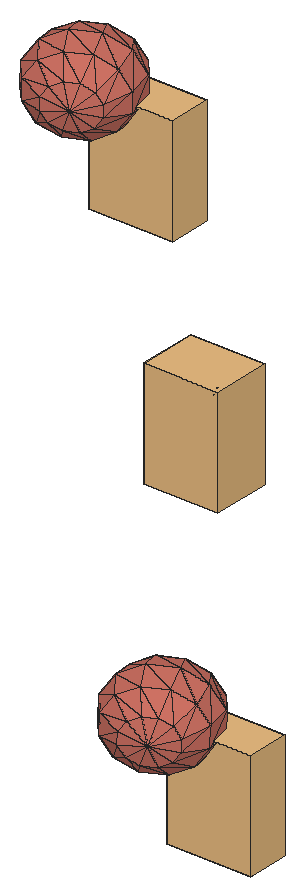
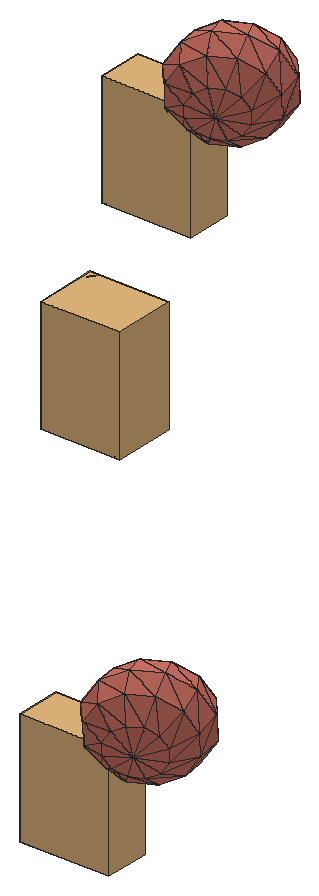
# SketchUp Ruby script. Lengths in inches.
U = 1.inch
M = Sketchup.active_model
def pt(a) = Geom::Point3d.new(a.map { |v| v * U })
def face(e, loops, mat)
  f = e.add_face(loops[0].map { |a| pt(a) })
  loops[1..].each { |l| e.add_face(l.map { |a| pt(a) }).erase! }
  f.material = f.back_material = mat if mat
  f
end
# faces: each face lists its corners as indices into pts; further lists are holes
def faces(e, pts, list, mat = nil) = list.each { |f| face(e, (f[0].is_a?(Array) ? f : [f]).map { |l| l.map { |i| pts[i] } }, mat) }
# xy, xz, yz: faces in a plane at the given z, y or x. An outline is a flat list of corners, or four numbers for a rectangle; further outlines are holes
def ring(l) = l.size == 4 ? [[l[0], l[1]], [l[2], l[1]], [l[2], l[3]], [l[0], l[3]]] : l.each_slice(2).to_a
def flat(e, list, mat, &to3) = list.each { |f| face(e, (f[0].is_a?(Array) ? f : [f]).map { |l| ring(l).map { |u, v| to3.(u, v) } }, mat) }
def xy(e, z, list, mat = nil) = flat(e, list, mat) { |x, y| [x, y, z] }
def xz(e, y, list, mat = nil) = flat(e, list, mat) { |x, z| [x, y, z] }
def yz(e, x, list, mat = nil) = flat(e, list, mat) { |y, z| [x, y, z] }
def lines(e, pts, list) = list.each { |a, b| e.add_line(pt(pts[a]), pt(pts[b])) }
# prism: a flat outline (further loops are holes) pulled along v
def prism(e, loops, v, mat = nil)
  f = face(e, loops, mat); d = Geom::Vector3d.new(v.map { |x| x * U })
  f.pushpull(f.normal.samedirection?(d) ? d.length : -d.length)
end
def box(e, o, s, mat = nil) = prism(e, [[o, [o[0] + s[0], o[1], o[2]], [o[0] + s[0], o[1] + s[1], o[2]], [o[0], o[1] + s[1], o[2]]]], [0, 0, s[2]], mat)
def at(x, y, z, deg = 0) = Geom::Transformation.translation(pt([x, y, z])) * Geom::Transformation.rotation(ORIGIN, Z_AXIS, deg.degrees)
def axes(o, x, y, z) = Geom::Transformation.new([*x, 0, *y, 0, *z, 0, *pt(o).to_a, 1])
def part(name) = M.definitions.add(name)
# library, detail: a bought-in or finely detailed component or shape, given as its bounding box
def library(name, o, s) = part(name).tap { |d| box(d.entities, o, s) }
def detail(e, o, s) = box(e.add_group.entities, o, s)
def put(e, d, t, mat = nil) = e.add_instance(d, t).tap { |i| i.material = mat if mat }
def group(e, t, mat = nil) = e.add_group.tap { |g| g.transformation = t; g.material = mat if mat }.entities
root = M.entities
M.materials.add("green").color = [174, 139, 102]
M.materials.add("vio").color = [206, 114, 100]
c1 = part("3DGeom~219_Defintion")
p = [[167.16,-297.35,-320.32],[-80.93,-262.73,-388.47],[-36.76,-95.49,-489.125],[218.17,-104.25,-436.54],[-281.83,-61.15,-410.64],[-43.21,95.93,-488.48],
  [-285.56,49.37,-410.27],[210.71,116.79,-435.8],[-317.52,144.24,-351.51],[-98.5625,260.26,-386.7],[-98.5625,260.26,-386.7],[370.46,-252.3,-166.34],
  [370.46,-252.3,-166.34],[414.63,-85.07,-266.99],[414.63,-85.07,-266.99],[414.63,-85.07,-266.99],[408.18,106.36,-266.34],[408.18,106.36,-266.34],
  [146.8,306.54,-318.28],[-98.5625,260.26,-386.7],[146.8,306.54,-318.28],[-307.34,-157.7,-352.53],[-281.83,-61.15,-410.64],[-307.34,-157.7,-352.53],
  [-451.39,-10.42,-222.13],[-285.56,49.37,-410.27],[-281.83,-61.15,-410.64],[-317.52,144.24,-351.51],[-285.56,49.37,-410.27],[71.36,-410.78,-118.27],
  [-163.89,-360.96,-213.49],[-80.93,-262.73,-388.47],[-80.93,-262.73,-388.47],[167.16,-297.35,-320.32],[-163.89,-360.96,-213.49],[-98.5625,260.26,-386.7],
  [-369.14,198.04,-250.11],[-98.5625,260.26,-386.7],[-369.14,198.04,-250.11],[-187.98,353.45,-211.07],[146.8,306.54,-318.28],[-98.5625,260.26,-386.7],
  [-187.98,353.45,-211.07],[-163.89,-360.96,-213.49],[-355.23,-214.42,-251.51],[-307.34,-157.7,-352.53],[-355.23,-214.42,-251.51],[-369.14,198.04,-250.11],
  [-317.52,144.24,-351.51],[287.5,-350.53,8.64],[167.16,-297.35,-320.32],[287.5,-350.53,8.64],[167.16,-297.35,-320.32],[370.46,-252.3,-166.34],
  [408.18,106.36,-266.34],[146.8,306.54,-318.28],[352.83,270.68,-164.57],[352.83,270.68,-164.57],[43.55,414.14,-115.47],[474.5,-139.65,32.21],
  [370.46,-252.3,-166.34],[414.63,-85.07,-266.99],[500,-43.09,-25.9],[408.18,106.36,-266.34],[496.27,67.43,-25.53],[352.83,270.68,-164.57],
  [-263.41,-363.87,-11.0625],[-412.69,-216.1,-134.63],[-355.23,-214.42,-251.51],[-355.23,-214.42,-251.51],[-355.23,-214.42,-251.51],[-412.69,-216.1,-134.63],
  [-426.6,196.36,-133.24],[-187.98,353.45,-211.07],[-412.69,-216.1,-134.63],[-464.32,-162.3,-33.23],[-496.27,-67.42,25.53],[-500,43.09,25.9],
  [-474.5,139.65,-32.21],[-43.55,-414.14,115.47],[-187.98,353.45,-211.07],[-287.5,350.54,-8.64],[-287.5,350.54,-8.64],[426.6,-196.36,133.24],
  [287.5,-350.53,8.64],[464.32,162.3,33.23],[263.41,363.87,11.0625],[352.83,270.68,-164.57],[263.41,363.87,11.0625],[-352.83,-270.68,164.57],
  [-412.69,-216.1,-134.63],[-263.41,-363.87,-11.0625],[-352.83,-270.68,164.57],[-412.69,-216.1,-134.63],[-287.5,350.54,-8.64],[187.98,-353.45,211.07],
  [187.98,-353.45,211.07],[287.5,-350.53,8.64],[-71.36,410.78,118.27],[-408.18,-106.36,266.34],[-352.83,-270.68,164.57],[-408.18,-106.36,266.34],
  [-370.46,252.3,166.34],[-287.5,350.54,-8.64],[-370.46,252.3,166.34],[451.39,10.42,222.13],[-146.8,-306.54,318.28],[-146.8,-306.54,318.28],
  [-352.83,-270.68,164.57],[-370.46,252.3,166.34],[369.14,-198.04,250.11],[187.98,-353.45,211.07],[263.41,363.87,11.0625],[412.69,216.1,134.63],
  [412.69,216.1,134.63],[163.89,360.96,213.49],[163.89,360.96,213.49],[-414.63,85.07,266.99],[-408.18,-106.36,266.34],[-414.63,85.07,266.99],
  [-370.46,252.3,166.34],[-414.63,85.07,266.99],[98.5625,-260.26,386.7],[-146.8,-306.54,318.28],[98.5625,-260.26,386.7],[187.98,-353.45,211.07],
  [-370.46,252.3,166.34],[-167.16,297.35,320.32],[163.89,360.96,213.49],[-167.16,297.35,320.32],[355.23,214.42,251.51],[412.69,216.1,134.63],
  [163.89,360.96,213.49],[355.23,214.42,251.51],[-210.71,-116.79,435.8],[-352.83,-270.68,164.57],[-146.8,-306.54,318.28],[-408.18,-106.36,266.34],
  [-167.16,297.35,320.32],[-370.46,252.3,166.34],[-414.63,85.07,266.99],[317.52,-144.24,351.51],[98.5625,-260.26,386.7],[187.98,-353.45,211.07],
  [317.52,-144.24,351.51],[187.98,-353.45,211.07],[369.14,-198.04,250.11],[355.23,214.42,251.51],[163.89,360.96,213.49],[80.93,262.73,388.47],
  [163.89,360.96,213.49],[-167.16,297.35,320.32],[80.93,262.73,388.47],[317.52,-144.24,351.51],[285.56,-49.37,410.27],[281.83,61.15,410.64],
  [307.34,157.7,352.53],[355.23,214.42,251.51],[307.34,157.7,352.53],[-218.17,104.25,436.54],[43.21,-95.93,488.48],[285.56,-49.37,410.27],
  [317.52,-144.24,351.51],[307.34,157.7,352.53],[36.76,95.49,489.125],[281.83,61.15,410.64],[307.34,157.7,352.53],[285.56,-49.37,410.27],
  [281.83,61.15,410.64],[285.56,-49.37,410.27],[281.83,61.15,410.64]]
faces(c1.entities,p,[[0,1,2],[0,2,3],[1,4,2],[3,2,5],[2,4,6],[2,6,5],[3,5,7],[5,6,8],
  [5,8,9],[7,5,10],[11,0,3],[12,3,13],[14,3,7],[15,7,16],[17,7,18],[7,19,20],
  [1,21,4],[22,23,24],[25,26,24],[27,28,24],[29,30,31],[29,32,33],[34,21,1],[35,8,36],
  [37,38,39],[40,41,42],[43,44,21],[45,46,24],[47,48,24],[49,29,50],[51,52,53],[54,55,56],
  [57,40,58],[40,42,58],[59,60,61],[59,61,62],[62,61,63],[62,63,64],[64,63,65],[66,67,68],
  [66,69,30],[70,71,24],[72,47,24],[73,47,72],[74,75,24],[75,76,24],[76,77,24],[77,78,24],
  [78,72,24],[79,66,30],[79,30,29],[80,72,81],[58,42,82],[83,84,60],[83,60,59],[64,65,85],
  [85,65,86],[87,58,88],[89,90,91],[92,75,93],[94,72,78],[95,79,29],[96,29,97],[58,82,98],
  [88,58,98],[99,75,100],[101,76,75],[102,78,77],[103,78,104],[59,62,105],[62,64,105],[64,85,105],
  [106,66,79],[107,108,66],[98,82,109],[110,111,84],[110,84,83],[85,112,113],[114,88,115],[88,98,116],
  [117,76,118],[119,77,76],[120,77,121],[83,59,105],[85,113,105],[122,123,79],[124,79,125],[98,126,127],
  [128,98,129],[110,83,105],[113,130,105],[131,132,133],[134,135,136],[134,137,135],[138,139,140],[141,142,143],
  [144,145,146],[147,148,149],[150,151,152],[153,110,105],[154,153,105],[155,154,105],[156,155,105],[130,156,105],
  [157,149,158],[159,137,134],[159,140,137],[138,140,159],[160,134,136],[160,136,142],[149,138,159],[161,142,162],
  [163,164,165],[166,149,164],[167,160,142],[149,159,164],[168,160,169],[170,164,160],[164,159,134],[164,134,160]],"vio")
c2 = library("3DGeom~96_Defintion",[-195.05,-500,-388.01],[390.1,1000,776.02])
c3 = part("3DGeom~97_Defintion")
p = [[174.48,487.39,-384.2],[155.8125,487.85,-388.01],[137.83,489.88,-382.14],[174.48,487.39,-384.2],[125.36,492.93,-368.18],[121.74,496.1875,-349.85],
  [174.48,487.39,-384.2],[121.74,496.1875,-349.85],[127.94,498.77,-332.09],[174.48,487.39,-384.2],[137.83,489.88,-382.14],[125.36,492.93,-368.18],
  [174.48,487.39,-384.2],[127.94,498.77,-332.09],[142.3,500,-319.63],[174.48,487.39,-384.2],[142.3,500,-319.63],[160.98,499.54,-315.83],
  [174.48,487.39,-384.2],[160.98,499.54,-315.83],[178.96,497.51,-321.7],[174.48,487.39,-384.2],[191.43,494.46,-335.66],[195.05,491.2,-353.98],
  [174.48,487.39,-384.2],[195.05,491.2,-353.98],[188.85,488.61,-371.75],[174.48,487.39,-384.2],[178.96,497.51,-321.7],[191.43,494.46,-335.66],
  [-147.29,-500,333.96],[-182.28,-490.37,332.19],[-165.51,-497.625,329.13],[-182.28,-490.37,332.19],[-147.29,-500,333.96],[-195.05,-469.79,356.79],
  [-182.28,-490.37,332.19],[-195.05,-469.79,356.79],[-193.09,-480.18,342.3125],[-195.05,-469.79,356.79],[-147.29,-500,333.96],[-172.82,-458.84,383.18],
  [-172.82,-458.84,383.18],[-147.29,-500,333.96],[-137.83,-468.47,384.95],[-147.29,-500,333.96],[-132.48,-496.86,345.39],[-125.0625,-489.05,360.34],
  [-137.83,-468.47,384.95],[-147.29,-500,333.96],[-125.0625,-489.05,360.34],[-195.05,-469.79,356.79],[-172.82,-458.84,383.18],[-187.63,-461.98,371.75],
  [-137.83,-468.47,384.95],[-125.0625,-489.05,360.34],[-127.02,-478.66,374.83],[-172.82,-458.84,383.18],[-137.83,-468.47,384.95],[-154.59,-461.21,388.01]]
faces(c3.entities,p,[[0,1,2],[3,4,5],[6,7,8],[9,10,11],[12,13,14],[15,16,17],[18,19,20],[21,22,23],
  [24,25,26],[27,28,29],[30,31,32],[33,34,35],[36,37,38],[39,40,41],[42,43,44],[45,46,47],
  [48,49,50],[51,52,53],[54,55,56],[57,58,59]],"green")
c4 = part("3DGeom~218_Defintion")
p = [[167.16,-297.35,-320.32],[-80.93,-262.73,-388.47],[-36.76,-95.49,-489.125],[218.17,-104.25,-436.54],[-281.83,-61.15,-410.64],[-43.21,95.93,-488.48],
  [-285.56,49.37,-410.27],[210.71,116.79,-435.8],[-317.52,144.24,-351.51],[-98.5625,260.26,-386.7],[-98.5625,260.26,-386.7],[370.46,-252.3,-166.34],
  [370.46,-252.3,-166.34],[414.63,-85.07,-266.99],[414.63,-85.07,-266.99],[414.63,-85.07,-266.99],[408.18,106.36,-266.34],[408.18,106.36,-266.34],
  [146.8,306.54,-318.28],[-98.5625,260.26,-386.7],[146.8,306.54,-318.28],[-307.34,-157.7,-352.53],[-281.83,-61.15,-410.64],[-307.34,-157.7,-352.53],
  [-451.39,-10.42,-222.13],[-285.56,49.37,-410.27],[-281.83,-61.15,-410.64],[-317.52,144.24,-351.51],[-285.56,49.37,-410.27],[71.36,-410.78,-118.27],
  [-163.89,-360.96,-213.49],[-80.93,-262.73,-388.47],[-80.93,-262.73,-388.47],[167.16,-297.35,-320.32],[-163.89,-360.96,-213.49],[-98.5625,260.26,-386.7],
  [-369.14,198.04,-250.11],[-98.5625,260.26,-386.7],[-369.14,198.04,-250.11],[-187.98,353.45,-211.07],[146.8,306.54,-318.28],[-98.5625,260.26,-386.7],
  [-187.98,353.45,-211.07],[-163.89,-360.96,-213.49],[-355.23,-214.42,-251.51],[-307.34,-157.7,-352.53],[-355.23,-214.42,-251.51],[-369.14,198.04,-250.11],
  [-317.52,144.24,-351.51],[287.5,-350.53,8.64],[167.16,-297.35,-320.32],[287.5,-350.53,8.64],[167.16,-297.35,-320.32],[370.46,-252.3,-166.34],
  [408.18,106.36,-266.34],[146.8,306.54,-318.28],[352.83,270.68,-164.57],[352.83,270.68,-164.57],[43.55,414.14,-115.47],[474.5,-139.65,32.21],
  [370.46,-252.3,-166.34],[414.63,-85.07,-266.99],[500,-43.09,-25.9],[408.18,106.36,-266.34],[496.27,67.43,-25.53],[352.83,270.68,-164.57],
  [-263.41,-363.87,-11.0625],[-412.69,-216.1,-134.63],[-355.23,-214.42,-251.51],[-355.23,-214.42,-251.51],[-355.23,-214.42,-251.51],[-412.69,-216.1,-134.63],
  [-426.6,196.36,-133.24],[-187.98,353.45,-211.07],[-412.69,-216.1,-134.63],[-464.32,-162.3,-33.23],[-496.27,-67.42,25.53],[-500,43.09,25.9],
  [-474.5,139.65,-32.21],[-43.55,-414.14,115.47],[-187.98,353.45,-211.07],[-287.5,350.54,-8.64],[-287.5,350.54,-8.64],[426.6,-196.36,133.24],
  [287.5,-350.53,8.64],[464.32,162.3,33.23],[263.41,363.87,11.0625],[352.83,270.68,-164.57],[263.41,363.87,11.0625],[-352.83,-270.68,164.57],
  [-412.69,-216.1,-134.63],[-263.41,-363.87,-11.0625],[-352.83,-270.68,164.57],[-412.69,-216.1,-134.63],[-287.5,350.54,-8.64],[187.98,-353.45,211.07],
  [187.98,-353.45,211.07],[287.5,-350.53,8.64],[-71.36,410.78,118.27],[-408.18,-106.36,266.34],[-352.83,-270.68,164.57],[-408.18,-106.36,266.34],
  [-370.46,252.3,166.34],[-287.5,350.54,-8.64],[-370.46,252.3,166.34],[451.39,10.42,222.13],[-146.8,-306.54,318.28],[-146.8,-306.54,318.28],
  [-352.83,-270.68,164.57],[-370.46,252.3,166.34],[369.14,-198.04,250.11],[187.98,-353.45,211.07],[263.41,363.87,11.0625],[412.69,216.1,134.63],
  [412.69,216.1,134.63],[163.89,360.96,213.49],[163.89,360.96,213.49],[-414.63,85.07,266.99],[-408.18,-106.36,266.34],[-414.63,85.07,266.99],
  [-370.46,252.3,166.34],[-414.63,85.07,266.99],[98.5625,-260.26,386.7],[-146.8,-306.54,318.28],[98.5625,-260.26,386.7],[187.98,-353.45,211.07],
  [-370.46,252.3,166.34],[-167.16,297.35,320.32],[163.89,360.96,213.49],[-167.16,297.35,320.32],[355.23,214.42,251.51],[412.69,216.1,134.63],
  [163.89,360.96,213.49],[355.23,214.42,251.51],[-210.71,-116.79,435.8],[-352.83,-270.68,164.57],[-146.8,-306.54,318.28],[-408.18,-106.36,266.34],
  [-167.16,297.35,320.32],[-370.46,252.3,166.34],[-414.63,85.07,266.99],[317.52,-144.24,351.51],[98.5625,-260.26,386.7],[187.98,-353.45,211.07],
  [317.52,-144.24,351.51],[187.98,-353.45,211.07],[369.14,-198.04,250.11],[355.23,214.42,251.51],[163.89,360.96,213.49],[80.93,262.73,388.47],
  [163.89,360.96,213.49],[-167.16,297.35,320.32],[80.93,262.73,388.47],[317.52,-144.24,351.51],[285.56,-49.37,410.27],[281.83,61.15,410.64],
  [307.34,157.7,352.53],[355.23,214.42,251.51],[307.34,157.7,352.53],[-218.17,104.25,436.54],[43.21,-95.93,488.48],[285.56,-49.37,410.27],
  [317.52,-144.24,351.51],[307.34,157.7,352.53],[36.76,95.49,489.125],[281.83,61.15,410.64],[307.34,157.7,352.53],[285.56,-49.37,410.27],
  [281.83,61.15,410.64],[285.56,-49.37,410.27],[281.83,61.15,410.64]]
faces(c4.entities,p,[[0,1,2],[0,2,3],[1,4,2],[3,2,5],[2,4,6],[2,6,5],[3,5,7],[5,6,8],
  [5,8,9],[7,5,10],[11,0,3],[12,3,13],[14,3,7],[15,7,16],[17,7,18],[7,19,20],
  [1,21,4],[22,23,24],[25,26,24],[27,28,24],[29,30,31],[29,32,33],[34,21,1],[35,8,36],
  [37,38,39],[40,41,42],[43,44,21],[45,46,24],[47,48,24],[49,29,50],[51,52,53],[54,55,56],
  [57,40,58],[40,42,58],[59,60,61],[59,61,62],[62,61,63],[62,63,64],[64,63,65],[66,67,68],
  [66,69,30],[70,71,24],[72,47,24],[73,47,72],[74,75,24],[75,76,24],[76,77,24],[77,78,24],
  [78,72,24],[79,66,30],[79,30,29],[80,72,81],[58,42,82],[83,84,60],[83,60,59],[64,65,85],
  [85,65,86],[87,58,88],[89,90,91],[92,75,93],[94,72,78],[95,79,29],[96,29,97],[58,82,98],
  [88,58,98],[99,75,100],[101,76,75],[102,78,77],[103,78,104],[59,62,105],[62,64,105],[64,85,105],
  [106,66,79],[107,108,66],[98,82,109],[110,111,84],[110,84,83],[85,112,113],[114,88,115],[88,98,116],
  [117,76,118],[119,77,76],[120,77,121],[83,59,105],[85,113,105],[122,123,79],[124,79,125],[98,126,127],
  [128,98,129],[110,83,105],[113,130,105],[131,132,133],[134,135,136],[134,137,135],[138,139,140],[141,142,143],
  [144,145,146],[147,148,149],[150,151,152],[153,110,105],[154,153,105],[155,154,105],[156,155,105],[130,156,105],
  [157,149,158],[159,137,134],[159,140,137],[138,140,159],[160,134,136],[160,136,142],[149,138,159],[161,142,162],
  [163,164,165],[166,149,164],[167,160,142],[149,159,164],[168,160,169],[170,164,160],[164,159,134],[164,134,160]],"vio")
c5 = library("3DGeom~94_Defintion",[-195.05,-500,-388.01],[390.1,1000,776.02])
c6 = part("3DGeom~95_Defintion")
p = [[174.48,487.39,-384.2],[155.8125,487.85,-388.01],[137.83,489.88,-382.14],[174.48,487.39,-384.2],[125.36,492.93,-368.18],[121.74,496.1875,-349.85],
  [174.48,487.39,-384.2],[121.74,496.1875,-349.85],[127.94,498.77,-332.09],[174.48,487.39,-384.2],[137.83,489.88,-382.14],[125.36,492.93,-368.18],
  [174.48,487.39,-384.2],[127.94,498.77,-332.09],[142.3,500,-319.63],[174.48,487.39,-384.2],[142.3,500,-319.63],[160.98,499.54,-315.83],
  [174.48,487.39,-384.2],[160.98,499.54,-315.83],[178.96,497.51,-321.7],[174.48,487.39,-384.2],[191.43,494.46,-335.66],[195.05,491.2,-353.98],
  [174.48,487.39,-384.2],[195.05,491.2,-353.98],[188.85,488.61,-371.75],[174.48,487.39,-384.2],[178.96,497.51,-321.7],[191.43,494.46,-335.66],
  [-147.28,-500,333.96],[-182.28,-490.37,332.19],[-165.51,-497.625,329.13],[-182.28,-490.37,332.19],[-147.28,-500,333.96],[-195.05,-469.79,356.79],
  [-182.28,-490.37,332.19],[-195.05,-469.79,356.79],[-193.09,-480.18,342.3125],[-195.05,-469.79,356.79],[-147.28,-500,333.96],[-172.82,-458.84,383.18],
  [-172.82,-458.84,383.18],[-147.28,-500,333.96],[-137.83,-468.47,384.95],[-147.28,-500,333.96],[-132.48,-496.86,345.39],[-125.06,-489.05,360.34],
  [-137.83,-468.47,384.95],[-147.28,-500,333.96],[-125.06,-489.05,360.34],[-195.05,-469.79,356.79],[-172.82,-458.84,383.18],[-187.63,-461.98,371.75],
  [-137.83,-468.47,384.95],[-125.06,-489.05,360.34],[-127.02,-478.66,374.83],[-172.82,-458.84,383.18],[-137.83,-468.47,384.95],[-154.59,-461.21,388.01]]
faces(c6.entities,p,[[0,1,2],[3,4,5],[6,7,8],[9,10,11],[12,13,14],[15,16,17],[18,19,20],[21,22,23],
  [24,25,26],[27,28,29],[30,31,32],[33,34,35],[36,37,38],[39,40,41],[42,43,44],[45,46,47],
  [48,49,50],[51,52,53],[54,55,56],[57,58,59]],"green")
c7 = library("3DGeom~74_Defintion",[-269.59,-500,-344.14],[539.17,1000,688.28])
c8 = part("3DGeom~75_Defintion")
p = [[-217.33,-469.79,-343.43],[-251.16,-458.84,-336.67],[-234.01,-461.98,-344.14],[-217.33,-469.79,-343.43],[-220.35,-500,-290.57],[-251.16,-458.84,-336.67],
  [-201.93,-490.37,-320.375],[-201.93,-490.37,-320.375],[-217.33,-469.79,-343.43],[-205.59,-480.18,-334.73],[-269.59,-468.47,-306.87],[-251.16,-458.84,-336.67],
  [-269.59,-468.47,-306.87],[-264.18,-461.21,-323.03],[-220.35,-500,-290.57],[-201.93,-490.37,-320.375],[-207.33,-497.625,-304.21],[-254.18,-489.05,-283.82],
  [-269.59,-468.47,-306.87],[-254.18,-489.05,-283.82],[-265.93,-478.66,-292.52],[-220.35,-500,-290.57],[-237.5,-496.86,-283.11],[-254.18,-489.05,-283.82],
  [253.72,487.39,337.56],[230.5,498.77,271.66],[212.66,500,278.24],[253.72,487.39,337.56],[249.06,496.1875,274.79],[230.5,498.77,271.66],
  [253.72,487.39,337.56],[263.36,492.93,286.79],[249.06,496.1875,274.79],[253.72,487.39,337.56],[212.66,500,278.24],[200.33,499.54,292.76],
  [253.72,487.39,337.56],[269.58,489.88,304.45],[263.36,492.93,286.79],[253.72,487.39,337.56],[200.33,499.54,292.76],[196.8,497.51,311.34],
  [253.72,487.39,337.56],[266.06,487.85,323.03],[269.58,489.88,304.45],[253.72,487.39,337.56],[196.8,497.51,311.34],[203.02,494.46,329],
  [253.72,487.39,337.56],[203.02,494.46,329],[217.33,491.2,341.01],[253.72,487.39,337.56],[217.33,491.2,341.01],[235.89,488.61,344.14]]
faces(c8.entities,p,[[0,1,2],[3,4,5],[6,4,3],[7,8,9],[5,4,10],[11,12,13],[14,15,16],[10,4,17],
  [18,19,20],[21,22,23],[24,25,26],[27,28,29],[30,31,32],[33,34,35],[36,37,38],[39,40,41],
  [42,43,44],[45,46,47],[48,49,50],[51,52,53]],"green")
g1 = group(root,at(15.3125,134.49,26.21))
put(g1,c1,axes([-2.11,-0.4,15.58],[0,0.00039,0],[0,0,-0.00039],[-0.00039,0,0]),"vio")
g2 = group(root,at(15.3125,134.49,26.21))
put(g2,c2,axes([-1.94,-0.32,15.36],[0,0.0004,0],[0,0,-0.0004],[-0.0004,0,0]),"green")
put(g2,c3,axes([-1.94,-0.32,15.36],[0,0.0004,0],[0,0,-0.0004],[-0.0004,0,0]),"green")
g3 = group(root,at(15.3125,134.49,26.21))
put(g3,c4,axes([-1.88,-0.33,13.53],[0,0.00039,0],[0,0,-0.00039],[-0.00039,0,0]),"vio")
g4 = group(root,at(15.3125,134.49,26.21))
put(g4,c5,axes([-1.71,-0.25,13.31],[0,0.0004,0],[0,0,-0.0004],[-0.0004,0,0]),"green")
put(g4,c6,axes([-1.71,-0.25,13.31],[0,0.0004,0],[0,0,-0.0004],[-0.0004,0,0]),"green")
g5 = group(root,at(15.3125,134.49,26.21))
put(g5,c7,axes([-1.7,-0.36,14.57],[0,0.0004,0],[0,0,-0.0004],[-0.0004,0,0]),"green")
put(g5,c8,axes([-1.7,-0.36,14.57],[0,0.0004,0],[0,0,-0.0004],[-0.0004,0,0]),"green")
